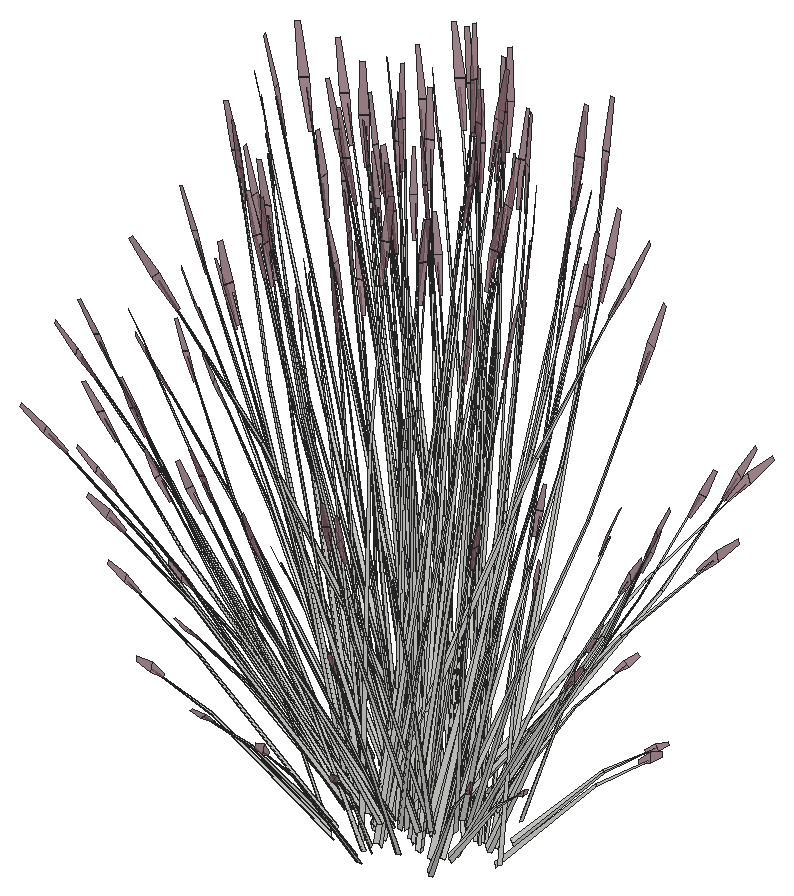
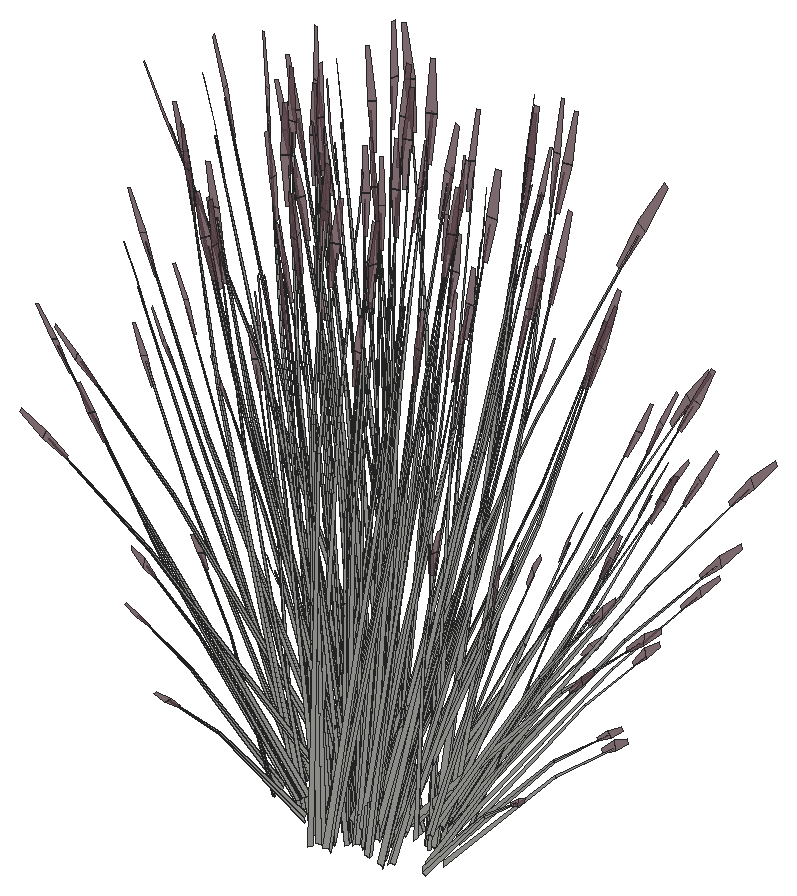
# SketchUp Ruby script. Lengths in millimetres.
U = 1.mm
M = Sketchup.active_model
def pt(a) = Geom::Point3d.new(a.map { |v| v * U })
def face(e, loops, mat)
  f = e.add_face(loops[0].map { |a| pt(a) })
  loops[1..].each { |l| e.add_face(l.map { |a| pt(a) }).erase! }
  f.material = f.back_material = mat if mat
  f
end
# faces: each face lists its corners as indices into pts; further lists are holes
def faces(e, pts, list, mat = nil) = list.each { |f| face(e, (f[0].is_a?(Array) ? f : [f]).map { |l| l.map { |i| pts[i] } }, mat) }
# xy, xz, yz: faces in a plane at the given z, y or x. An outline is a flat list of corners, or four numbers for a rectangle; further outlines are holes
def ring(l) = l.size == 4 ? [[l[0], l[1]], [l[2], l[1]], [l[2], l[3]], [l[0], l[3]]] : l.each_slice(2).to_a
def flat(e, list, mat, &to3) = list.each { |f| face(e, (f[0].is_a?(Array) ? f : [f]).map { |l| ring(l).map { |u, v| to3.(u, v) } }, mat) }
def xy(e, z, list, mat = nil) = flat(e, list, mat) { |x, y| [x, y, z] }
def xz(e, y, list, mat = nil) = flat(e, list, mat) { |x, z| [x, y, z] }
def yz(e, x, list, mat = nil) = flat(e, list, mat) { |y, z| [x, y, z] }
def lines(e, pts, list) = list.each { |a, b| e.add_line(pt(pts[a]), pt(pts[b])) }
# prism: a flat outline (further loops are holes) pulled along v
def prism(e, loops, v, mat = nil)
  f = face(e, loops, mat); d = Geom::Vector3d.new(v.map { |x| x * U })
  f.pushpull(f.normal.samedirection?(d) ? d.length : -d.length)
end
def box(e, o, s, mat = nil) = prism(e, [[o, [o[0] + s[0], o[1], o[2]], [o[0] + s[0], o[1] + s[1], o[2]], [o[0], o[1] + s[1], o[2]]]], [0, 0, s[2]], mat)
def at(x, y, z, deg = 0) = Geom::Transformation.translation(pt([x, y, z])) * Geom::Transformation.rotation(ORIGIN, Z_AXIS, deg.degrees)
def axes(o, x, y, z) = Geom::Transformation.new([*x, 0, *y, 0, *z, 0, *pt(o).to_a, 1])
def part(name) = M.definitions.add(name)
# library, detail: a bought-in or finely detailed component or shape, given as its bounding box
def library(name, o, s) = part(name).tap { |d| box(d.entities, o, s) }
def detail(e, o, s) = box(e.add_group.entities, o, s)
def put(e, d, t, mat = nil) = e.add_instance(d, t).tap { |i| i.material = mat if mat }
def group(e, t, mat = nil) = e.add_group.tap { |g| g.transformation = t; g.material = mat if mat }.entities
root = M.entities
M.materials.add("LightPink_Translucent").color = [144, 107, 117]
M.materials["LightPink_Translucent"].alpha = 0.8
c1 = part("blade")
p = [[54.7,5.3,558.8],[0,4.4,0],[2.3,11.5,0],[55.5,7.8,558.8],[58.2,7.8,558.8],[9.8,11.5,0],
  [62.9,5.7,838.2],[63,6,838.2],[63.4,6,838.2]]
faces(c1.entities,p,[[0,1,2,3],[4,5,2,3],[6,0,3,7],[7,3,4,8]])
c2 = part("seeds")
p = [[7.6,-2.7,35.1],[-0.2,-0.6,40.4],[-0.2,-0.8,0.9],[3.5,-1.8,-1.7],[7.5,-0.8,76.3],[3.7,0.2,78.9]]
faces(c2.entities,p,[[0,1,2,3],[1,0,4,5]],"LightPink_Translucent")
c3 = part("blade with seeds")
put(c3.entities,c1,at(0,0,0))
put(c3.entities,c2,axes([60.9,6.5,787.2],[1.5799,-0.05474,1.17369],[-0.12525,1.92788,0.29478],[-0.07173,-0.02425,1.56792]))
put(root,c3,axes([14033.3,4330.2,8503],[0.50831,-0.02346,1.71376],[-0.33721,1.01661,0.13857],[-0.72439,-0.06288,0.73262]))
put(root,c3,axes([14038.7,4375.7,8503],[0.42521,-0.21906,1.71376],[0.35798,1.01226,0.13857],[-0.66754,0.22878,0.73262]))
put(root,c3,axes([14005,4419.5,8470.3],[0.42589,0.08502,1.43002],[0.2745,0.86839,-0.30754],[-0.57851,0.16255,0.61141]))
put(root,c3,axes([14100.7,4348.8,8489.4],[0.34834,-0.14982,1.77064],[0.12012,1.04605,0.13857],[-0.75452,0.1388,0.63284]))
put(root,c3,axes([14071.9,4306.2,8531],[-1.22504,-0.02494,-0.71045],[0.08228,-1.05005,0.08574],[-0.51899,-0.11081,1.00501]))
put(root,c3,axes([14046.8,4312.7,8470.3],[0.23927,0.28834,1.43002],[-0.55135,0.78376,-0.30754],[-0.56612,-0.18733,0.61141]))
put(root,c3,axes([14021.9,4352.4,8519.5],[-1.01846,-0.28891,-0.35414],[0.29705,-0.84289,0.4572],[-0.41005,0.07729,0.87481]))
put(root,c3,axes([14057.7,4288.8,8503],[0.45521,0.17844,1.71376],[-0.94204,0.74856,0.13857],[-0.58713,-0.33769,0.73262]))
put(root,c3,axes([14039.7,4363.3,8523.4],[-0.332,0.94205,-0.51099],[-1.13828,-0.3229,-0.3958],[-0.45829,0.08638,0.97773]))
put(root,c3,axes([14061.6,4311.6,8523.4],[-0.88986,0.68603,-0.51099],[-0.77932,-0.72471,-0.3958],[-0.45212,-0.10438,0.97773]))
put(root,c3,axes([14025.1,4361.8,8442.4],[0.03108,0.16322,1.76342],[-0.62654,0.85237,-0.26939],[-0.44504,-0.04296,0.30037]))
put(root,c3,axes([13982.5,4465.7,8474.7],[0.51072,-0.46938,1.1486],[0.20153,0.74307,0.84392],[-0.36908,0.13305,0.25299]))
put(root,c3,axes([14053.2,4295.2,8519.5],[-0.69728,-0.64842,-0.35414],[0.79619,-0.61382,0.4572],[-0.40453,-0.09339,0.87481]))
put(root,c3,axes([14078.2,4393,8503],[0.30609,-0.31822,1.71376],[0.77286,0.85893,0.13857],[-0.53009,0.39116,0.73262]))
put(root,c3,axes([14031.4,4414.1,8519.5],[-1.06674,0.14801,-0.35414],[-0.28168,-0.84611,0.4572],[-0.30569,0.22726,0.87481]))
put(root,c3,axes([14010.7,4334.7,8474.7],[0.78239,-0.07411,1.1486],[-0.49629,0.65296,0.84392],[-0.38663,-0.09795,0.25299]))
put(root,c3,axes([14053.7,4416.7,8523.4],[0.31482,0.94565,-0.51099],[-1.19224,0.16542,-0.3958],[-0.34166,0.254,0.97773]))
put(root,c3,axes([14129.2,4399.4,8456.8],[-1.27479,-0.1698,-0.62353],[0.26901,-1.04736,-0.16365],[-0.38043,-0.12691,1.37633]))
put(root,c3,axes([14126,4274.8,8531],[-1.04497,-0.50058,-0.71045],[0.74264,-0.8772,0.08574],[-0.3786,-0.29889,1.00501]))
put(root,c3,axes([14113.6,4275.4,8523.4],[-1.20928,0.24619,-0.51099],[-0.21154,-0.93233,-0.3958],[-0.32481,-0.26718,0.97773]))
put(root,c3,axes([14086.7,4449.8,8455.8],[-1.14694,-0.51783,-0.49651],[0.68554,-0.92854,0],[-0.26122,-0.11794,1.57504]))
put(root,c3,axes([14074,4253.9,8442.4],[-0.11871,0.13643,1.76342],[-1.19964,0.29415,-0.26939],[-0.2898,-0.26759,0.30037]))
put(root,c3,axes([14104.5,4465.6,8464.8],[-0.7662,1.03778,0],[-1.28187,-0.57875,-0.51607],[-0.29196,-0.13181,1.63711]))
put(root,c3,axes([14055,4267.2,8458.6],[-0.35352,0.84566,-0.03893],[-1.08806,-0.26014,-0.17649],[-0.1652,-0.13832,0.58215]))
put(root,c3,axes([14096.3,4240.1,8470.3],[-0.07421,0.33879,1.43002],[-1.08488,0.28361,-0.30754],[-0.25359,-0.4379,0.61141]))
put(root,c3,axes([14105.3,4262.4,8503],[0.28013,0.33252,1.71376],[-1.29445,0.27994,0.13857],[-0.29256,-0.52202,0.73262]))
put(root,c3,axes([14166,4403.4,8472.2],[-1.23732,0.68758,-0.29095],[-0.8228,-0.97154,-0.50002],[-0.30528,-0.09867,1.59708]))
put(root,c3,axes([14116.8,4258,8519.5],[-0.18927,-0.83419,-0.35414],[1.08199,-0.22027,0.4572],[-0.29062,-0.23905,0.87481]))
put(root,c3,axes([14040.2,4365.3,8464.8],[-1.53239,0,0],[0,-1.1575,-0.51607],[0,-0.26363,1.63711]))
put(root,c3,axes([14094.9,4440,8456],[-0.28787,-0.90242,-0.30978],[1.14332,-0.25625,0.30978],[-0.23049,-0.10406,1.38974]))
put(root,c3,axes([14186.8,4422.4,8456.8],[-0.82544,0.77843,-0.62353],[-1.0254,-0.70586,-0.16365],[-0.33076,0.19418,1.37633]))
put(root,c3,axes([14070.3,4357.5,8463.7],[-1.1399,0.87071,0.30756],[-1.1406,-0.86155,-0.36492],[-0.03981,-0.24727,1.64885]))
put(root,c3,axes([14189.5,4418.6,8489],[1.05902,0.41762,1.51261],[-1.03748,0.89969,0.59816],[-0.46471,-0.53324,1.26806]))
put(root,c3,axes([14086.8,4226.3,8474.7],[0.63926,0.36046,1.1486],[-0.93099,0.21668,0.84392],[-0.1992,-0.27702,0.25299]))
put(root,c3,axes([14201.3,4411.3,8467.1],[-1.19666,-0.83357,-0.25192],[1.00694,-0.93603,0.5513],[-0.32224,0.09751,1.68216]))
put(root,c3,axes([14146,4391,8460.7],[-0.73619,-0.86927,-0.44739],[1.11511,-0.61213,0.21531],[-0.23824,-0.10756,1.43643]))
put(root,c3,axes([14185.9,4406.8,8460.7],[-1.33077,0.06393,-0.44739],[-0.12035,-1.06125,0.21531],[-0.23824,0.10756,1.43643]))
put(root,c3,axes([14121.3,4451.9,8467.5],[1.14694,0.51783,0.49651],[-0.68554,0.92854,0],[-0.26122,-0.11794,1.57504]))
put(root,c3,axes([14148.7,4403.6,8466.5],[0.32481,-1.2272,-0.23429],[1.54007,0.21392,0.51271],[-0.26911,-0.16947,1.5644]))
put(root,c3,axes([14163,4411,8471],[-0.23642,0.92427,0.1448],[-1.15506,-0.16044,-0.41347],[-0.21021,-0.09491,1.26744]))
put(root,c3,axes([14221.4,4476.4,8455.8],[-1.14694,0.51783,-0.49651],[-0.68554,-0.92854,0],[-0.26122,0.11794,1.57504]))
put(root,c3,axes([14048.9,4345.3,8455.8],[0,-1.03566,-0.49651],[1.37109,0,0],[0,-0.23588,1.57504]))
put(root,c3,axes([14063.8,4369.7,8467.5],[0,1.03566,0.49651],[-1.37109,0,0],[0,-0.23588,1.57504]))
put(root,c3,axes([14223.3,4469.3,8460.2],[-0.75665,-1.04141,-0.05142],[1.28187,-0.57875,0.51607],[-0.31588,0.09915,1.6363]))
put(root,c3,axes([14214.5,4466,8456],[-1.14332,-0.25625,-0.30978],[0.28787,-0.90242,0.30978],[-0.23049,0.10406,1.38974]))
put(root,c3,axes([14139.9,4375.7,8472.2],[-1.38012,-0.49416,-0.29095],[0.66454,-1.04299,-0.50002],[-0.04337,-0.25608,1.59708]))
put(root,c3,axes([14209.6,4399.5,8472.2],[0.1428,1.18174,-0.29095],[-1.48733,0.07145,-0.50002],[-0.26191,0.15741,1.59708]))
put(root,c3,axes([14124.2,4349.1,8457.8],[-0.50328,-1.06202,-0.69835],[1.44974,-0.38248,-0.18329],[-0.05563,-0.35963,1.54149]))
put(root,c3,axes([14181.8,4264.4,8523.4],[-1.20468,-0.25962,-0.51099],[0.41292,-0.89013,-0.3958],[-0.11046,-0.35838,0.97773]))
put(root,c3,axes([14063.8,4345.9,8456],[0.85545,-0.64616,-0.30978],[0.85545,0.64616,0.30978],[0,-0.20813,1.38974]))
put(root,c3,axes([14161.9,4239.8,8458.6],[-0.84686,0.59414,-0.03893],[-0.77596,-0.65071,-0.17649],[-0.05463,-0.18438,0.58215]))
put(root,c3,axes([14153.3,4388.6,8464.5],[1.54892,0.2182,0.45755],[-0.31522,1.23236,0.17955],[-0.22636,-0.119,1.58856]))
put(root,c3,axes([14143.1,4382.9,8473.6],[-0.59459,0.93321,0.44739],[-1.23546,-0.44912,-0.21531],[0,-0.21512,1.43643]))
put(root,c3,axes([14192.9,4268.7,8531],[-0.5849,-0.8421,-0.71045],[1.20401,-0.4693,0.08574],[-0.13677,-0.40688,1.00501]))
put(root,c3,axes([14132.2,4438.6,8467.4],[1.31687,-0.27488,0.17642],[0.32517,1.02297,0.35086],[-0.11745,-0.14905,1.60407]))
put(root,c3,axes([14175.2,4442.7,8460.3],[-1.23546,-0.46496,0],[0.59459,-0.96613,0],[0,0,1.62707]))
put(root,c3,axes([14247.8,4472.3,8464.8],[0.7662,1.03778,0],[-1.28187,0.57875,-0.51607],[-0.29196,0.13181,1.63711]))
put(root,c3,axes([14231.7,4440,8467.4],[0.35402,-1.02926,0.17642],[1.29548,0.29127,0.35086],[-0.22379,0.00501,1.60407]))
put(root,c3,axes([14216.5,4405.3,8471],[0.90538,0.62224,0.1448],[-0.75521,0.70202,-0.41347],[-0.21021,0.09491,1.26744]))
put(root,c3,axes([14208.3,4385.8,8462.9],[-1.1399,-0.8914,-0.06131],[1.1406,-0.89194,0],[-0.03981,-0.03113,1.75571]))
put(root,c3,axes([14215.9,4393.8,8473.6],[1.33077,-0.06393,0.44739],[0.12035,1.06125,-0.21531],[-0.23824,0.10756,1.43643]))
put(root,c3,axes([14224.2,4455.7,8463.7],[1.53422,0.33662,0.30756],[-0.38383,1.20322,-0.36492],[-0.25393,0.15059,1.64885]))
put(root,c3,axes([14167.3,4221.3,8442.4],[-0.20555,0.03731,1.76342],[-1.13672,-0.42002,-0.26939],[0.01907,-0.35034,0.30037]))
put(root,c3,axes([14241,4454,8467.5],[1.14694,-0.51783,0.49651],[0.68554,0.92854,0],[-0.26122,0.11794,1.57504]))
put(root,c3,axes([14195.8,4250.6,8519.5],[0.36946,-0.79643,-0.35414],[1.07787,0.23229,0.4572],[-0.09883,-0.32066,0.87481]))
put(root,c3,axes([14149.9,4359.8,8464.5],[0.53281,1.15808,0.45755],[-1.52239,0.4027,0.17955],[0.01861,-0.2128,1.58856]))
put(root,c3,axes([14143.7,4356,8460.7],[0.59459,-0.93321,-0.44739],[1.23546,0.44912,0.21531],[0,-0.21512,1.43643]))
put(root,c3,axes([14182.4,4432.5,8460.5],[-0.39985,-0.89288,0],[1.1418,-0.31268,0],[0,0,1.54371]))
put(root,c3,axes([14223.3,4387.8,8460.7],[-0.59459,0.93321,-0.44739],[-1.23546,-0.44912,0.21531],[0,0.21512,1.43643]))
put(root,c3,axes([14283.1,4373.3,8467.4],[-0.96285,-0.75439,0.17642],[0.97031,-0.7317,0.35086],[-0.10634,0.15406,1.60407]))
put(root,c3,axes([14198.6,4362.3,8460.5],[0,-1.19833,0],[1.53239,0,0],[0,0,1.79456]))
put(root,c3,axes([14162.4,4367.8,8466.3],[1.3808,0.50196,0.24065],[-0.66454,1.04299,0.50002],[0,-0.24043,1.60543]))
put(root,c3,axes([14218.1,4374.4,8462.7],[0,1.19774,-0.05637],[-1.53239,0,0],[0,0.03764,1.79368]))
put(root,c3,axes([14151.1,4350.1,8473.6],[-1.33077,0.06393,0.44739],[-0.12035,-1.06125,-0.21531],[0.23824,-0.10756,1.43643]))
put(root,c3,axes([14135.3,4303.8,8467.4],[-0.35402,1.02926,0.17642],[-1.29548,-0.29127,0.35086],[0.22379,-0.00501,1.60407]))
put(root,c3,axes([14199.5,4433.3,8462.7],[0.53281,1.18979,-0.06012],[-1.52239,0.41691,0],[0.01861,0.04155,1.72173]))
put(root,c3,axes([14119.2,4271.5,8464.8],[-0.7662,-1.03778,0],[1.28187,-0.57875,-0.51607],[0.29196,-0.13181,1.63711]))
put(root,c3,axes([14311.3,4393.7,8460.4],[-1.53164,-0.00828,-0.04976],[0,-1.1575,0.49943],[-0.04813,0.2635,1.58352]))
put(root,c3,axes([14234.9,4305.2,8467.4],[-1.31687,0.27488,0.17642],[-0.32517,-1.02297,0.35086],[0.11745,0.14905,1.60407]))
put(root,c3,axes([14200.7,4207.8,8474.7],[0.15721,0.60392,1.1486],[-0.87211,-0.33448,0.84392],[0.09385,-0.30923,0.25299]))
put(root,c3,axes([14180.1,4343.1,8464.5],[-1.01611,0.93987,0.45755],[-1.20717,-0.82966,0.17955],[0.24496,-0.0938,1.58856]))
put(root,c3,axes([14224.2,4380.7,8460.8],[0.85545,0.66896,0],[-0.85545,0.66896,0],[0,0,1.69266]))
put(root,c3,axes([14223.9,4360.9,8473.6],[0.59459,-0.93321,0.44739],[1.23546,0.44912,-0.21531],[0,0.21512,1.43643]))
put(root,c3,axes([14210.8,4443.2,8460.5],[1.23546,0.46496,0],[-0.59459,0.96613,0],[0,0,1.74954]))
put(root,c3,axes([14213.7,4355.2,8465],[-1.54892,-0.2182,0.49198],[0.31522,-1.23236,0.19306],[0.22636,0.119,1.70813]))
put(root,c3,axes([14303.2,4397.9,8456],[-0.85545,0.64616,-0.30978],[-0.85545,-0.64616,0.30978],[0,0.20813,1.38974]))
put(root,c3,axes([14225,4369.1,8460.5],[1.37109,0,0],[0,1.07219,0],[0,0,1.78407]))
put(root,c3,axes([14191.5,4339,8473.6],[-0.73619,-0.86927,0.44739],[1.11511,-0.61213,-0.21531],[0.23824,0.10756,1.43643]))
put(root,c3,axes([14157.5,4344.3,8472.2],[-0.1428,-1.18174,-0.29095],[1.48733,-0.07145,-0.50002],[0.26191,-0.15741,1.59708]))
put(root,c3,axes([14237,4366.3,8471],[1.1418,-0.30203,0.1448],[0.39985,0.86246,-0.41347],[0,0.18981,1.26744]))
put(root,c3,axes([14247.9,4281.6,8523.4],[-0.87728,-0.69587,-0.51099],[0.92674,-0.60943,-0.3958],[0.13348,-0.35356,0.97773]))
put(root,c3,axes([14227.1,4368.1,8472.2],[1.38012,0.49416,-0.29095],[-0.66454,1.04299,-0.50002],[0.04337,0.25608,1.59708]))
put(root,c3,axes([14152.5,4277.8,8456],[1.14332,0.25625,-0.30978],[-0.28787,0.90242,0.30978],[0.23049,-0.10406,1.38974]))
put(root,c3,axes([14233.3,4250.2,8470.3],[-0.34835,0.20963,1.43002],[-1.04325,-0.36691,-0.30754],[0.19338,-0.4563,0.61141]))
put(root,c3,axes([14303.2,4374.1,8467.5],[0,-1.03566,0.49651],[1.37109,0,0],[0,0.23588,1.57504]))
put(root,c3,axes([14318.1,4398.5,8455.8],[0,1.03566,-0.49651],[-1.37109,0,0],[0,0.23588,1.57504]))
put(root,c3,axes([14145.7,4267.4,8455.8],[1.14694,-0.51783,-0.49651],[0.68554,0.92854,0],[0.26122,-0.11794,1.57504]))
put(root,c3,axes([14204,4332.8,8471],[0.23642,-0.92427,0.1448],[1.15506,0.16044,-0.41347],[0.21021,0.09491,1.26744]))
put(root,c3,axes([14245.8,4291.9,8467.5],[-1.14694,-0.51783,0.49651],[0.68554,-0.92854,0],[0.26122,0.11794,1.57504]))
put(root,c3,axes([14254.8,4289.7,8531],[0.03189,-0.95798,-0.71045],[1.34277,0.06434,0.08574],[0.14171,-0.40585,1.00501]))
put(root,c3,axes([14220.4,4429.3,8460],[1.2866,-0.3514,-0.19198],[0.45209,1.01223,0.00008],[0.14202,-0.03884,1.73897]))
put(root,c3,axes([14221,4352.9,8460.7],[0.73619,0.86927,-0.44739],[-1.11511,0.61213,0.21531],[0.23824,0.10756,1.43643]))
put(root,c3,axes([14268.9,4275,8519.5],[0.82919,-0.54528,-0.35414],[0.78493,0.62262,0.4572],[0.11943,-0.31634,0.87481]))
put(root,c3,axes([14273.9,4453.1,8474.7],[-0.69001,-0.29779,1.1486],[0.89096,-0.30257,0.84392],[0.24031,0.2563,0.25299]))
put(root,c3,axes([14180.2,4321.4,8456.8],[0.82544,-0.77843,-0.62353],[1.0254,0.70586,-0.16365],[0.33076,-0.19418,1.37633]))
put(root,c3,axes([14272.2,4303.9,8456],[0.28787,0.90242,-0.30978],[-1.14332,0.25625,0.30978],[0.23049,0.10406,1.38974]))
put(root,c3,axes([14326.8,4378.6,8464.9],[1.53239,0,0],[0,1.1575,-0.51607],[0,0.26363,1.63711]))
put(root,c3,axes([14201.1,4340.5,8472.2],[1.23732,-0.68758,-0.29095],[0.8228,0.97154,-0.50002],[0.30528,0.09867,1.59708]))
put(root,c3,axes([14216.4,4277.3,8503],[-0.22818,0.35597,1.71376],[-0.95725,-0.73667,0.13857],[0.43183,-0.45914,0.73262]))
put(root,c3,axes([14121.7,4324.9,8445],[-1.20625,0.41464,1.28929],[-0.38394,-1.1897,0.50096],[0.74071,0.01979,1.46642]))
put(root,c3,axes([14262.5,4278.2,8464.9],[0.7662,-1.03778,0],[1.28187,0.57875,-0.51607],[0.29196,0.13181,1.63711]))
put(root,c3,axes([14295.1,4266.6,8442.4],[-0.18342,-0.08159,1.76342],[-0.47115,-0.9115,-0.26939],[0.31784,-0.24736,0.30037]))
put(root,c3,axes([14280.3,4294,8455.8],[1.14694,0.51783,-0.49651],[-0.68554,0.92854,0],[0.26122,0.11794,1.57504]))
put(root,c3,axes([14294.2,4322.3,8523.4],[-0.31482,-0.94565,-0.51099],[1.19224,-0.16542,-0.3958],[0.34166,-0.254,0.97773]))
put(root,c3,axes([14347.4,4446.2,8504.3],[-0.23455,-0.87059,-0.03492],[1.10861,-0.20015,-0.15832],[0.23151,0.05519,0.52218]))
put(root,c3,axes([14237.8,4344.4,8456.8],[1.27479,0.1698,-0.62353],[-0.26901,1.04736,-0.16365],[0.38043,0.12691,1.37633]))
put(root,c3,axes([14375.6,4360.1,8461.9],[-0.75977,-0.66224,-0.06488],[0.83212,-0.6068,-0.29416],[0.23578,-0.04272,0.97024]))
put(root,c3,axes([14331.3,4274.5,8474.7],[-0.40819,0.5272,1.1486],[-0.35086,-0.70831,0.84392],[0.33713,-0.17749,0.25299]))
put(root,c3,axes([14231.1,4401.5,8503],[-0.45521,-0.17844,1.71376],[0.94204,-0.74856,0.13857],[0.58713,0.33769,0.73262]))
put(root,c3,axes([14316.5,4324.8,8519.5],[1.06674,-0.14801,-0.35414],[0.28168,0.84611,0.4572],[0.30569,-0.22726,0.87481]))
put(root,c3,axes([14295,4332,8531],[0.64013,-0.81717,-0.71045],[1.12174,0.58074,0.08574],[0.38221,-0.29607,1.00501]))
put(root,c3,axes([14294.7,4443.7,8519.5],[0.69728,0.64842,-0.35414],[-0.79619,0.61382,0.4572],[0.40453,0.09339,0.87481]))
put(root,c3,axes([14308.3,4375.6,8523.4],[0.332,-0.94205,-0.51099],[1.13828,0.3229,-0.3958],[0.45829,-0.08638,0.97773]))
put(root,c3,axes([14380.9,4390.9,8474.7],[-0.75718,0.17097,1.1486],[0.35641,-0.70661,0.84392],[0.40168,0.04835,0.25299]))
put(root,c3,axes([14318.5,4312.9,8470.3],[-0.4378,-0.03068,1.43002],[-0.44851,-0.8229,-0.30754],[0.53783,-0.23279,0.61141]))
put(root,c3,axes([14326,4386.5,8519.5],[1.01846,0.28891,-0.35414],[-0.29705,0.84289,0.4572],[0.41005,-0.07729,0.87481]))
put(root,c3,axes([14276,4432.7,8531],[1.22504,0.02494,-0.71045],[-0.08228,1.05005,0.08574],[0.51899,0.11081,1.00501]))
put(root,c3,axes([14339.1,4382.3,8454.9],[-0.7893,0.12429,1.41583],[-0.12563,-0.9893,0.08104],[0.55282,-0.14974,0.80566]))
put(root,c3,axes([14361,4365.9,8442.4],[-0.06405,-0.15723,1.76342],[0.44421,-0.91974,-0.26939],[0.4481,-0.01323,0.30037]))
put(root,c3,axes([14255.5,4360,8503],[-0.50831,0.02346,1.71376],[0.33721,-1.01661,0.13857],[0.72439,0.06288,0.73262]))
put(root,c3,axes([14302.8,4384.3,8531],[1.07686,-0.45739,-0.71045],[0.60013,0.94154,0.08574],[0.52031,-0.10696,1.00501]))
